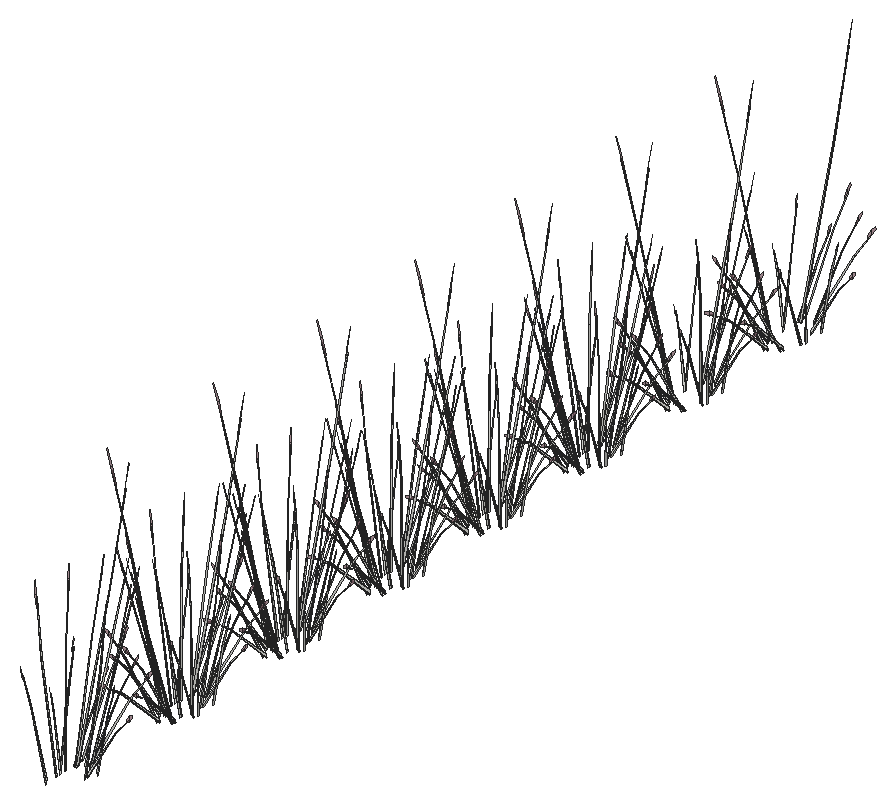
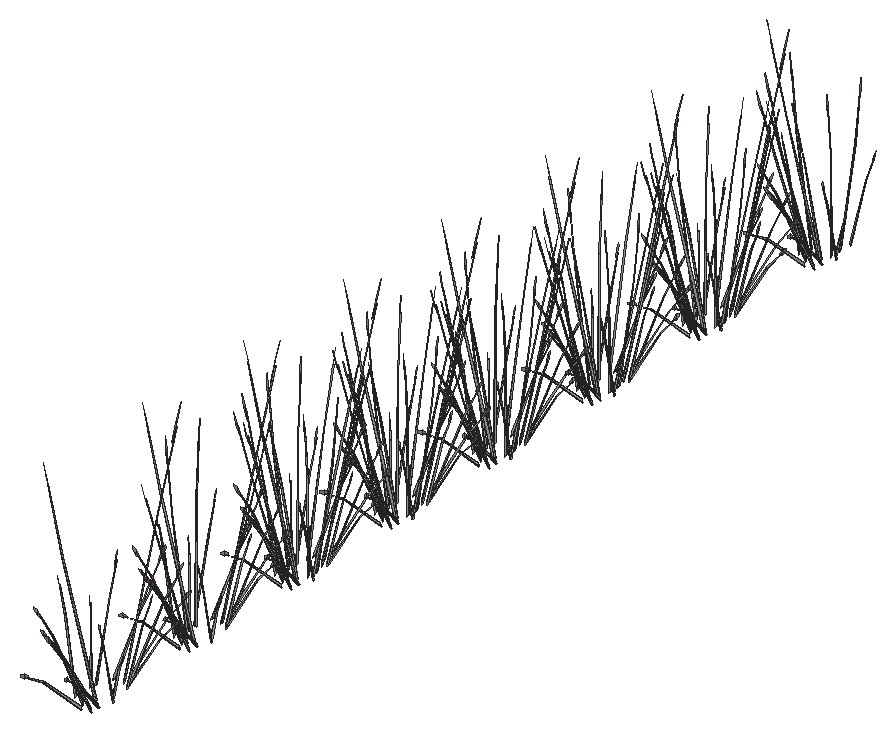
# SketchUp Ruby script. Lengths in inches.
U = 1.inch
M = Sketchup.active_model
def pt(a) = Geom::Point3d.new(a.map { |v| v * U })
def face(e, loops, mat)
  f = e.add_face(loops[0].map { |a| pt(a) })
  loops[1..].each { |l| e.add_face(l.map { |a| pt(a) }).erase! }
  f.material = f.back_material = mat if mat
  f
end
# faces: each face lists its corners as indices into pts; further lists are holes
def faces(e, pts, list, mat = nil) = list.each { |f| face(e, (f[0].is_a?(Array) ? f : [f]).map { |l| l.map { |i| pts[i] } }, mat) }
# xy, xz, yz: faces in a plane at the given z, y or x. An outline is a flat list of corners, or four numbers for a rectangle; further outlines are holes
def ring(l) = l.size == 4 ? [[l[0], l[1]], [l[2], l[1]], [l[2], l[3]], [l[0], l[3]]] : l.each_slice(2).to_a
def flat(e, list, mat, &to3) = list.each { |f| face(e, (f[0].is_a?(Array) ? f : [f]).map { |l| ring(l).map { |u, v| to3.(u, v) } }, mat) }
def xy(e, z, list, mat = nil) = flat(e, list, mat) { |x, y| [x, y, z] }
def xz(e, y, list, mat = nil) = flat(e, list, mat) { |x, z| [x, y, z] }
def yz(e, x, list, mat = nil) = flat(e, list, mat) { |y, z| [x, y, z] }
def lines(e, pts, list) = list.each { |a, b| e.add_line(pt(pts[a]), pt(pts[b])) }
# prism: a flat outline (further loops are holes) pulled along v
def prism(e, loops, v, mat = nil)
  f = face(e, loops, mat); d = Geom::Vector3d.new(v.map { |x| x * U })
  f.pushpull(f.normal.samedirection?(d) ? d.length : -d.length)
end
def box(e, o, s, mat = nil) = prism(e, [[o, [o[0] + s[0], o[1], o[2]], [o[0] + s[0], o[1] + s[1], o[2]], [o[0], o[1] + s[1], o[2]]]], [0, 0, s[2]], mat)
def at(x, y, z, deg = 0) = Geom::Transformation.translation(pt([x, y, z])) * Geom::Transformation.rotation(ORIGIN, Z_AXIS, deg.degrees)
def axes(o, x, y, z) = Geom::Transformation.new([*x, 0, *y, 0, *z, 0, *pt(o).to_a, 1])
def part(name) = M.definitions.add(name)
# library, detail: a bought-in or finely detailed component or shape, given as its bounding box
def library(name, o, s) = part(name).tap { |d| box(d.entities, o, s) }
def detail(e, o, s) = box(e.add_group.entities, o, s)
def put(e, d, t, mat = nil) = e.add_instance(d, t).tap { |i| i.material = mat if mat }
def group(e, t, mat = nil) = e.add_group.tap { |g| g.transformation = t; g.material = mat if mat }.entities
root = M.entities
M.materials.add("LightPink_Translucent").color = [144, 107, 117]
M.materials["LightPink_Translucent"].alpha = 0.75
c1 = part("blade")
p = [[2.15,0.21,22],[0,0.17,0],[0.09,0.45,0],[2.18,0.31,22],[2.29,0.31,22],[0.38,0.45,0],
  [2.48,0.24,33],[2.49,0.24,33],[2.48,0.22,33]]
faces(c1.entities,p,[[0,1,2,3],[4,5,2,3],[6,3,4,7],[8,0,3,6]])
c2 = part("seeds")
p = [[0.3,-0.1,1.38],[-0.01,-0.03,1.59],[-0.01,-0.03,0.03],[0.14,-0.07,-0.07],[0.29,-0.03,3],[0.15,0.01,3.11]]
faces(c2.entities,p,[[0,1,2,3],[1,0,4,5]],"LightPink_Translucent")
c3 = part("blade with seeds")
put(c3.entities,c1,at(0,0,0))
put(c3.entities,c2,axes([2.4,0.25,30.99],[1.5799,-0.05474,1.17369],[-0.12525,1.92788,0.29478],[-0.07173,-0.02425,1.56792]))
put(root,c3,axes([250.48,129.89,2.61],[0.01898,0.06102,1.28742],[-0.09148,0.54852,-0.12165],[-0.09264,0.00397,0.22783]))
put(root,c3,axes([250.44,131.76,2.625],[-0.09401,-0.41691,0.04667],[0.17143,-0.20406,0.3674],[-0.07557,0.04026,0.56022]))
put(root,c3,axes([252.88,132.97,2.625],[0.09401,0.41691,0.04667],[-0.17143,0.20406,0.3674],[0.07557,-0.04026,0.56022]))
put(root,c3,axes([253.29,134.63,2.61],[-0.02314,-0.05353,1.28742],[0.05063,-0.5738,-0.12165],[0.09117,-0.03666,0.22783]))
put(root,c3,axes([250.28,132.3,2.61],[-0.0418,0.07939,1.26972],[0.00356,0.58003,-0.2008],[-0.09581,0.07543,0.10183]))
put(root,c3,axes([252.72,133.76,2.61],[0.05491,-0.01034,1.26972],[0.1506,-0.47504,-0.2008],[0.09767,0.06271,0.10183]))
put(root,c3,axes([250.47,133.1875,2.625],[-0.17571,-0.25715,0.04667],[0.1023,-0.3662,0.3674],[-0.05634,0.11839,0.56022]))
put(root,c3,axes([249.81,132.89,2.61],[0.03267,0.0164,1.28742],[0.10105,0.54025,-0.12165],[-0.06687,0.1418,0.22783]))
put(root,c3,axes([252.58,134.24,2.625],[-0.01289,0.46496,0.04667],[-0.19462,-0.01275,0.3674],[0.07455,0.04865,0.56022]))
put(root,c3,axes([251.78,135.24,2.61],[0.00076,-0.07403,1.28742],[0.21935,-0.3266,-0.12165],[0.07619,0.11658,0.22783]))
put(root,c3,axes([250.82,134.4,2.625],[-0.21034,-0.02849,0.04667],[0.00577,-0.43021,0.3674],[-0.02201,0.1648,0.56022]))
put(root,c3,axes([252.04,135,2.625],[-0.11633,0.38842,0.04667],[-0.16566,-0.22614,0.3674],[0.05356,0.12453,0.56022]))
put(root,c3,axes([251.39,135.06,2.625],[-0.1886,0.20781,0.04667],[-0.09231,-0.37894,0.3674],[0.01821,0.16704,0.56022]))
put(root,c3,axes([250.29,134.46,2.61],[-0.00636,0.121,1.26972],[0.18056,0.42094,-0.2008],[-0.04727,0.19906,0.10183]))
put(root,c3,axes([250.86,134.19,3.11],[0.2813,0.0303,-0.09797],[-0.00769,0.57361,-0.54375],[-0.01954,0.22092,0.82622]))
put(root,c3,axes([250.27,135.71,2.61],[0.02904,-0.03692,1.28742],[0.24001,0.24555,-0.12165],[-0.00564,0.20445,0.22783]))
put(root,c3,axes([251.32,135.96,2.61],[0.03244,0.09846,1.26972],[0.26183,0.03868,-0.2008],[0.02633,0.21715,0.10183]))
put(root,c3,axes([251.55,146.22,2.61],[-0.03915,-0.08573,1.26972],[-0.26126,0.05435,-0.2008],[-0.0417,-0.20505,0.10183]))
put(root,c3,axes([252.72,147.27,2.61],[-0.00247,-0.12169,1.26972],[-0.20868,-0.35171,-0.2008],[0.03226,-0.2132,0.10183]))
put(root,c3,axes([252.66,146.83,2.61],[-0.02599,0.0467,1.28742],[-0.25468,-0.15757,-0.12165],[-0.00922,-0.20381,0.22783]))
put(root,c3,axes([251.28,145.9375,2.61],[-0.00478,0.07329,1.28742],[-0.23551,0.26599,-0.12165],[-0.0693,-0.13596,0.22783]))
put(root,c3,axes([251.9375,147.3125,2.625],[0.1886,-0.20781,0.04667],[0.09231,0.37894,0.3674],[-0.01821,-0.16704,0.56022]))
put(root,c3,axes([251.29,147.37,2.625],[0.11633,-0.38842,0.04667],[0.16566,0.22614,0.3674],[-0.05356,-0.12453,0.56022]))
put(root,c3,axes([251.34,147.33,3.13],[-0.17082,0.58618,-0.09885],[-0.24738,-0.33771,-0.54865],[-0.08599,-0.16561,0.83366]))
put(root,c3,axes([252.51,147.98,2.625],[0.21034,0.02849,0.04667],[-0.00577,0.43021,0.3674],[0.02201,-0.1648,0.56022]))
put(root,c3,axes([250.6875,147.16,2.61],[-0.05507,-0.00432,1.26972],[-0.17533,0.4316,-0.2008],[-0.09355,-0.08819,0.10183]))
put(root,c3,axes([253.35,149.16,2.61],[-0.03343,-0.00464,1.28742],[-0.13883,-0.49759,-0.12165],[0.05575,-0.16361,0.22783]))
put(root,c3,axes([250.75,148.14,2.625],[0.01289,-0.46496,0.04667],[0.19462,0.01275,0.3674],[-0.07455,-0.04865,0.56022]))
put(root,c3,axes([252.86,149.19,2.625],[0.17571,0.25715,0.04667],[-0.1023,0.3662,0.3674],[0.05634,-0.11839,0.56022]))
put(root,c3,axes([253.48,149.76,2.61],[0.03552,-0.09314,1.26972],[-0.04546,-0.57131,-0.2008],[0.08912,-0.10832,0.10183]))
put(root,c3,axes([250.48,147.53,2.61],[0.01898,0.06102,1.28742],[-0.09148,0.54852,-0.12165],[-0.09264,0.00397,0.22783]))
put(root,c3,axes([250.44,149.4,2.625],[-0.09401,-0.41691,0.04667],[0.17143,-0.20406,0.3674],[-0.07557,0.04026,0.56022]))
put(root,c3,axes([252.88,150.61,2.625],[0.09401,0.41691,0.04667],[-0.17143,0.20406,0.3674],[0.07557,-0.04026,0.56022]))
put(root,c3,axes([253.29,152.27,2.61],[-0.02314,-0.05353,1.28742],[0.05063,-0.5738,-0.12165],[0.09117,-0.03666,0.22783]))
put(root,c3,axes([250.28,149.94,2.61],[-0.0418,0.07939,1.26972],[0.00356,0.58003,-0.2008],[-0.09581,0.07543,0.10183]))
put(root,c3,axes([252.72,151.4,2.61],[0.05491,-0.01034,1.26972],[0.1506,-0.47504,-0.2008],[0.09767,0.06271,0.10183]))
put(root,c3,axes([250.47,150.83,2.625],[-0.17571,-0.25715,0.04667],[0.1023,-0.3662,0.3674],[-0.05634,0.11839,0.56022]))
put(root,c3,axes([249.81,150.53,2.61],[0.03267,0.0164,1.28742],[0.10105,0.54025,-0.12165],[-0.06687,0.1418,0.22783]))
put(root,c3,axes([252.58,151.88,2.625],[-0.01289,0.46496,0.04667],[-0.19462,-0.01275,0.3674],[0.07455,0.04865,0.56022]))
put(root,c3,axes([251.78,152.89,2.61],[0.00076,-0.07403,1.28742],[0.21935,-0.3266,-0.12165],[0.07619,0.11658,0.22783]))
put(root,c3,axes([250.82,152.04,2.625],[-0.21034,-0.02849,0.04667],[0.00577,-0.43021,0.3674],[-0.02201,0.1648,0.56022]))
put(root,c3,axes([252.04,152.64,2.625],[-0.11633,0.38842,0.04667],[-0.16566,-0.22614,0.3674],[0.05356,0.12453,0.56022]))
put(root,c3,axes([251.39,152.7,2.625],[-0.1886,0.20781,0.04667],[-0.09231,-0.37894,0.3674],[0.01821,0.16704,0.56022]))
put(root,c3,axes([250.29,152.11,2.61],[-0.00636,0.121,1.26972],[0.18056,0.42094,-0.2008],[-0.04727,0.19906,0.10183]))
put(root,c3,axes([250.86,151.83,3.11],[0.2813,0.0303,-0.09797],[-0.00769,0.57361,-0.54375],[-0.01954,0.22092,0.82622]))
put(root,c3,axes([250.27,153.35,2.61],[0.02904,-0.03692,1.28742],[0.24001,0.24555,-0.12165],[-0.00564,0.20445,0.22783]))
put(root,c3,axes([251.32,153.6,2.61],[0.03244,0.09846,1.26972],[0.26183,0.03868,-0.2008],[0.02633,0.21715,0.10183]))
put(root,c3,axes([251.55,162.49,2.61],[-0.03915,-0.08573,1.26972],[-0.26126,0.05435,-0.2008],[-0.0417,-0.20505,0.10183]))
put(root,c3,axes([252.72,163.54,2.61],[-0.00247,-0.12169,1.26972],[-0.20868,-0.35171,-0.2008],[0.03226,-0.2132,0.10183]))
put(root,c3,axes([252.66,163.1,2.61],[-0.02599,0.0467,1.28742],[-0.25468,-0.15757,-0.12165],[-0.00922,-0.20381,0.22783]))
put(root,c3,axes([251.28,162.21,2.61],[-0.00478,0.07329,1.28742],[-0.23551,0.26599,-0.12165],[-0.0693,-0.13596,0.22783]))
put(root,c3,axes([251.9375,163.58,2.625],[0.1886,-0.20781,0.04667],[0.09231,0.37894,0.3674],[-0.01821,-0.16704,0.56022]))
put(root,c3,axes([251.29,163.64,2.625],[0.11633,-0.38842,0.04667],[0.16566,0.22614,0.3674],[-0.05356,-0.12453,0.56022]))
put(root,c3,axes([251.34,163.6,3.13],[-0.17082,0.58618,-0.09885],[-0.24738,-0.33771,-0.54865],[-0.08599,-0.16561,0.83366]))
put(root,c3,axes([252.51,164.25,2.625],[0.21034,0.02849,0.04667],[-0.00577,0.43021,0.3674],[0.02201,-0.1648,0.56022]))
put(root,c3,axes([250.6875,163.43,2.61],[-0.05507,-0.00432,1.26972],[-0.17533,0.4316,-0.2008],[-0.09355,-0.08819,0.10183]))
put(root,c3,axes([253.35,165.43,2.61],[-0.03343,-0.00464,1.28742],[-0.13883,-0.49759,-0.12165],[0.05575,-0.16361,0.22783]))
put(root,c3,axes([250.75,164.41,2.625],[0.01289,-0.46496,0.04667],[0.19462,0.01275,0.3674],[-0.07455,-0.04865,0.56022]))
put(root,c3,axes([252.86,165.46,2.625],[0.17571,0.25715,0.04667],[-0.1023,0.3662,0.3674],[0.05634,-0.11839,0.56022]))
put(root,c3,axes([253.48,166.03,2.61],[0.03552,-0.09314,1.26972],[-0.04546,-0.57131,-0.2008],[0.08912,-0.10832,0.10183]))
put(root,c3,axes([250.48,163.8,2.61],[0.01898,0.06102,1.28742],[-0.09148,0.54852,-0.12165],[-0.09264,0.00397,0.22783]))
put(root,c3,axes([250.44,165.67,2.625],[-0.09401,-0.41691,0.04667],[0.17143,-0.20406,0.3674],[-0.07557,0.04026,0.56022]))
put(root,c3,axes([252.88,166.88,2.625],[0.09401,0.41691,0.04667],[-0.17143,0.20406,0.3674],[0.07557,-0.04026,0.56022]))
put(root,c3,axes([253.29,168.54,2.61],[-0.02314,-0.05353,1.28742],[0.05063,-0.5738,-0.12165],[0.09117,-0.03666,0.22783]))
put(root,c3,axes([250.28,166.21,2.61],[-0.0418,0.07939,1.26972],[0.00356,0.58003,-0.2008],[-0.09581,0.07543,0.10183]))
put(root,c3,axes([252.72,167.67,2.61],[0.05491,-0.01034,1.26972],[0.1506,-0.47504,-0.2008],[0.09767,0.06271,0.10183]))
put(root,c3,axes([250.47,167.1,2.625],[-0.17571,-0.25715,0.04667],[0.1023,-0.3662,0.3674],[-0.05634,0.11839,0.56022]))
put(root,c3,axes([249.81,166.8,2.61],[0.03267,0.0164,1.28742],[0.10105,0.54025,-0.12165],[-0.06687,0.1418,0.22783]))
put(root,c3,axes([252.58,168.15,2.625],[-0.01289,0.46496,0.04667],[-0.19462,-0.01275,0.3674],[0.07455,0.04865,0.56022]))
put(root,c3,axes([251.78,169.16,2.61],[0.00076,-0.07403,1.28742],[0.21935,-0.3266,-0.12165],[0.07619,0.11658,0.22783]))
put(root,c3,axes([250.82,168.31,2.625],[-0.21034,-0.02849,0.04667],[0.00577,-0.43021,0.3674],[-0.02201,0.1648,0.56022]))
put(root,c3,axes([252.04,168.91,2.625],[-0.11633,0.38842,0.04667],[-0.16566,-0.22614,0.3674],[0.05356,0.12453,0.56022]))
put(root,c3,axes([251.39,168.97,2.625],[-0.1886,0.20781,0.04667],[-0.09231,-0.37894,0.3674],[0.01821,0.16704,0.56022]))
put(root,c3,axes([250.29,168.38,2.61],[-0.00636,0.121,1.26972],[0.18056,0.42094,-0.2008],[-0.04727,0.19906,0.10183]))
put(root,c3,axes([250.86,168.1,3.11],[0.2813,0.0303,-0.09797],[-0.00769,0.57361,-0.54375],[-0.01954,0.22092,0.82622]))
put(root,c3,axes([250.27,169.62,2.61],[0.02904,-0.03692,1.28742],[0.24001,0.24555,-0.12165],[-0.00564,0.20445,0.22783]))
put(root,c3,axes([251.32,169.875,2.61],[0.03244,0.09846,1.26972],[0.26183,0.03868,-0.2008],[0.02633,0.21715,0.10183]))
put(root,c3,axes([251.55,178.34,2.61],[-0.03915,-0.08573,1.26972],[-0.26126,0.05435,-0.2008],[-0.0417,-0.20505,0.10183]))
put(root,c3,axes([252.72,179.39,2.61],[-0.00247,-0.12169,1.26972],[-0.20868,-0.35171,-0.2008],[0.03226,-0.2132,0.10183]))
put(root,c3,axes([252.66,178.95,2.61],[-0.02599,0.0467,1.28742],[-0.25468,-0.15757,-0.12165],[-0.00922,-0.20381,0.22783]))
put(root,c3,axes([251.28,178.06,2.61],[-0.00478,0.07329,1.28742],[-0.23551,0.26599,-0.12165],[-0.0693,-0.13596,0.22783]))
put(root,c3,axes([251.9375,179.43,2.625],[0.1886,-0.20781,0.04667],[0.09231,0.37894,0.3674],[-0.01821,-0.16704,0.56022]))
put(root,c3,axes([251.29,179.49,2.625],[0.11633,-0.38842,0.04667],[0.16566,0.22614,0.3674],[-0.05356,-0.12453,0.56022]))
put(root,c3,axes([251.34,179.45,3.13],[-0.17082,0.58618,-0.09885],[-0.24738,-0.33771,-0.54865],[-0.08599,-0.16561,0.83366]))
put(root,c3,axes([252.51,180.1,2.625],[0.21034,0.02849,0.04667],[-0.00577,0.43021,0.3674],[0.02201,-0.1648,0.56022]))
put(root,c3,axes([250.6875,179.28,2.61],[-0.05507,-0.00432,1.26972],[-0.17533,0.4316,-0.2008],[-0.09355,-0.08819,0.10183]))
put(root,c3,axes([253.35,181.28,2.61],[-0.03343,-0.00464,1.28742],[-0.13883,-0.49759,-0.12165],[0.05575,-0.16361,0.22783]))
put(root,c3,axes([250.75,180.26,2.625],[0.01289,-0.46496,0.04667],[0.19462,0.01275,0.3674],[-0.07455,-0.04865,0.56022]))
put(root,c3,axes([252.86,181.31,2.625],[0.17571,0.25715,0.04667],[-0.1023,0.3662,0.3674],[0.05634,-0.11839,0.56022]))
put(root,c3,axes([253.48,181.88,2.61],[0.03552,-0.09314,1.26972],[-0.04546,-0.57131,-0.2008],[0.08912,-0.10832,0.10183]))
put(root,c3,axes([250.48,179.65,2.61],[0.01898,0.06102,1.28742],[-0.09148,0.54852,-0.12165],[-0.09264,0.00397,0.22783]))
put(root,c3,axes([250.44,181.52,2.625],[-0.09401,-0.41691,0.04667],[0.17143,-0.20406,0.3674],[-0.07557,0.04026,0.56022]))
put(root,c3,axes([252.88,182.73,2.625],[0.09401,0.41691,0.04667],[-0.17143,0.20406,0.3674],[0.07557,-0.04026,0.56022]))
put(root,c3,axes([253.29,184.39,2.61],[-0.02314,-0.05353,1.28742],[0.05063,-0.5738,-0.12165],[0.09117,-0.03666,0.22783]))
put(root,c3,axes([250.28,182.0625,2.61],[-0.0418,0.07939,1.26972],[0.00356,0.58003,-0.2008],[-0.09581,0.07543,0.10183]))
put(root,c3,axes([252.72,183.52,2.61],[0.05491,-0.01034,1.26972],[0.1506,-0.47504,-0.2008],[0.09767,0.06271,0.10183]))
put(root,c3,axes([250.47,182.95,2.625],[-0.17571,-0.25715,0.04667],[0.1023,-0.3662,0.3674],[-0.05634,0.11839,0.56022]))
put(root,c3,axes([249.81,182.65,2.61],[0.03267,0.0164,1.28742],[0.10105,0.54025,-0.12165],[-0.06687,0.1418,0.22783]))
put(root,c3,axes([252.58,184,2.625],[-0.01289,0.46496,0.04667],[-0.19462,-0.01275,0.3674],[0.07455,0.04865,0.56022]))
put(root,c3,axes([251.78,185.01,2.61],[0.00076,-0.07403,1.28742],[0.21935,-0.3266,-0.12165],[0.07619,0.11658,0.22783]))
put(root,c3,axes([250.82,184.16,2.625],[-0.21034,-0.02849,0.04667],[0.00577,-0.43021,0.3674],[-0.02201,0.1648,0.56022]))
put(root,c3,axes([252.04,184.77,2.625],[-0.11633,0.38842,0.04667],[-0.16566,-0.22614,0.3674],[0.05356,0.12453,0.56022]))
put(root,c3,axes([251.39,184.82,2.625],[-0.1886,0.20781,0.04667],[-0.09231,-0.37894,0.3674],[0.01821,0.16704,0.56022]))
put(root,c3,axes([250.29,184.23,2.61],[-0.00636,0.121,1.26972],[0.18056,0.42094,-0.2008],[-0.04727,0.19906,0.10183]))
put(root,c3,axes([250.86,183.96,3.11],[0.2813,0.0303,-0.09797],[-0.00769,0.57361,-0.54375],[-0.01954,0.22092,0.82622]))
put(root,c3,axes([250.27,185.47,2.61],[0.02904,-0.03692,1.28742],[0.24001,0.24555,-0.12165],[-0.00564,0.20445,0.22783]))
put(root,c3,axes([251.55,193.33,2.61],[-0.03915,-0.08573,1.26972],[-0.26126,0.05435,-0.2008],[-0.0417,-0.20505,0.10183]))
put(root,c3,axes([251.32,185.73,2.61],[0.03244,0.09846,1.26972],[0.26183,0.03868,-0.2008],[0.02633,0.21715,0.10183]))
put(root,c3,axes([252.72,194.375,2.61],[-0.00247,-0.12169,1.26972],[-0.20868,-0.35171,-0.2008],[0.03226,-0.2132,0.10183]))
put(root,c3,axes([252.66,193.94,2.61],[-0.02599,0.0467,1.28742],[-0.25468,-0.15757,-0.12165],[-0.00922,-0.20381,0.22783]))
put(root,c3,axes([251.28,193.04,2.61],[-0.00478,0.07329,1.28742],[-0.23551,0.26599,-0.12165],[-0.0693,-0.13596,0.22783]))
put(root,c3,axes([251.9375,194.42,2.625],[0.1886,-0.20781,0.04667],[0.09231,0.37894,0.3674],[-0.01821,-0.16704,0.56022]))
put(root,c3,axes([251.29,194.48,2.625],[0.11633,-0.38842,0.04667],[0.16566,0.22614,0.3674],[-0.05356,-0.12453,0.56022]))
put(root,c3,axes([251.34,194.4375,3.13],[-0.17082,0.58618,-0.09885],[-0.24738,-0.33771,-0.54865],[-0.08599,-0.16561,0.83366]))
put(root,c3,axes([252.51,195.08,2.625],[0.21034,0.02849,0.04667],[-0.00577,0.43021,0.3674],[0.02201,-0.1648,0.56022]))
put(root,c3,axes([250.6875,194.27,2.61],[-0.05507,-0.00432,1.26972],[-0.17533,0.4316,-0.2008],[-0.09355,-0.08819,0.10183]))
put(root,c3,axes([253.35,196.27,2.61],[-0.03343,-0.00464,1.28742],[-0.13883,-0.49759,-0.12165],[0.05575,-0.16361,0.22783]))
put(root,c3,axes([250.75,195.24,2.625],[0.01289,-0.46496,0.04667],[0.19462,0.01275,0.3674],[-0.07455,-0.04865,0.56022]))
put(root,c3,axes([252.86,196.29,2.625],[0.17571,0.25715,0.04667],[-0.1023,0.3662,0.3674],[0.05634,-0.11839,0.56022]))
put(root,c3,axes([253.48,196.87,2.61],[0.03552,-0.09314,1.26972],[-0.04546,-0.57131,-0.2008],[0.08912,-0.10832,0.10183]))
put(root,c3,axes([250.48,194.64,2.61],[0.01898,0.06102,1.28742],[-0.09148,0.54852,-0.12165],[-0.09264,0.00397,0.22783]))
put(root,c3,axes([250.44,196.51,2.625],[-0.09401,-0.41691,0.04667],[0.17143,-0.20406,0.3674],[-0.07557,0.04026,0.56022]))
put(root,c3,axes([252.88,197.72,2.625],[0.09401,0.41691,0.04667],[-0.17143,0.20406,0.3674],[0.07557,-0.04026,0.56022]))
put(root,c3,axes([253.29,199.38,2.61],[-0.02314,-0.05353,1.28742],[0.05063,-0.5738,-0.12165],[0.09117,-0.03666,0.22783]))
put(root,c3,axes([250.28,197.05,2.61],[-0.0418,0.07939,1.26972],[0.00356,0.58003,-0.2008],[-0.09581,0.07543,0.10183]))
put(root,c3,axes([252.72,198.51,2.61],[0.05491,-0.01034,1.26972],[0.1506,-0.47504,-0.2008],[0.09767,0.06271,0.10183]))
put(root,c3,axes([250.47,197.9375,2.625],[-0.17571,-0.25715,0.04667],[0.1023,-0.3662,0.3674],[-0.05634,0.11839,0.56022]))
put(root,c3,axes([249.81,197.64,2.61],[0.03267,0.0164,1.28742],[0.10105,0.54025,-0.12165],[-0.06687,0.1418,0.22783]))
put(root,c3,axes([252.58,198.99,2.625],[-0.01289,0.46496,0.04667],[-0.19462,-0.01275,0.3674],[0.07455,0.04865,0.56022]))
put(root,c3,axes([251.78,199.99,2.61],[0.00076,-0.07403,1.28742],[0.21935,-0.3266,-0.12165],[0.07619,0.11658,0.22783]))
put(root,c3,axes([250.82,199.15,2.625],[-0.21034,-0.02849,0.04667],[0.00577,-0.43021,0.3674],[-0.02201,0.1648,0.56022]))
put(root,c3,axes([252.04,199.75,2.625],[-0.11633,0.38842,0.04667],[-0.16566,-0.22614,0.3674],[0.05356,0.12453,0.56022]))
put(root,c3,axes([251.39,199.81,2.625],[-0.1886,0.20781,0.04667],[-0.09231,-0.37894,0.3674],[0.01821,0.16704,0.56022]))
put(root,c3,axes([250.29,199.21,2.61],[-0.00636,0.121,1.26972],[0.18056,0.42094,-0.2008],[-0.04727,0.19906,0.10183]))
put(root,c3,axes([250.86,198.94,3.11],[0.2813,0.0303,-0.09797],[-0.00769,0.57361,-0.54375],[-0.01954,0.22092,0.82622]))
put(root,c3,axes([250.27,200.46,2.61],[0.02904,-0.03692,1.28742],[0.24001,0.24555,-0.12165],[-0.00564,0.20445,0.22783]))
put(root,c3,axes([251.55,208.58,2.61],[-0.03915,-0.08573,1.26972],[-0.26126,0.05435,-0.2008],[-0.0417,-0.20505,0.10183]))
put(root,c3,axes([251.32,200.71,2.61],[0.03244,0.09846,1.26972],[0.26183,0.03868,-0.2008],[0.02633,0.21715,0.10183]))
put(root,c3,axes([252.72,209.63,2.61],[-0.00247,-0.12169,1.26972],[-0.20868,-0.35171,-0.2008],[0.03226,-0.2132,0.10183]))
put(root,c3,axes([252.66,209.19,2.61],[-0.02599,0.0467,1.28742],[-0.25468,-0.15757,-0.12165],[-0.00922,-0.20381,0.22783]))
put(root,c3,axes([251.28,208.3,2.61],[-0.00478,0.07329,1.28742],[-0.23551,0.26599,-0.12165],[-0.0693,-0.13596,0.22783]))
put(root,c3,axes([251.9375,209.67,2.625],[0.1886,-0.20781,0.04667],[0.09231,0.37894,0.3674],[-0.01821,-0.16704,0.56022]))
put(root,c3,axes([251.29,209.73,2.625],[0.11633,-0.38842,0.04667],[0.16566,0.22614,0.3674],[-0.05356,-0.12453,0.56022]))
put(root,c3,axes([251.34,209.69,3.13],[-0.17082,0.58618,-0.09885],[-0.24738,-0.33771,-0.54865],[-0.08599,-0.16561,0.83366]))
put(root,c3,axes([252.51,210.34,2.625],[0.21034,0.02849,0.04667],[-0.00577,0.43021,0.3674],[0.02201,-0.1648,0.56022]))
put(root,c3,axes([250.6875,209.52,2.61],[-0.05507,-0.00432,1.26972],[-0.17533,0.4316,-0.2008],[-0.09355,-0.08819,0.10183]))
put(root,c3,axes([253.35,211.52,2.61],[-0.03343,-0.00464,1.28742],[-0.13883,-0.49759,-0.12165],[0.05575,-0.16361,0.22783]))
put(root,c3,axes([250.75,210.5,2.625],[0.01289,-0.46496,0.04667],[0.19462,0.01275,0.3674],[-0.07455,-0.04865,0.56022]))
put(root,c3,axes([252.86,211.55,2.625],[0.17571,0.25715,0.04667],[-0.1023,0.3662,0.3674],[0.05634,-0.11839,0.56022]))
put(root,c3,axes([253.48,212.12,2.61],[0.03552,-0.09314,1.26972],[-0.04546,-0.57131,-0.2008],[0.08912,-0.10832,0.10183]))
put(root,c3,axes([250.48,209.89,2.61],[0.01898,0.06102,1.28742],[-0.09148,0.54852,-0.12165],[-0.09264,0.00397,0.22783]))
put(root,c3,axes([250.44,211.76,2.625],[-0.09401,-0.41691,0.04667],[0.17143,-0.20406,0.3674],[-0.07557,0.04026,0.56022]))
put(root,c3,axes([252.88,212.97,2.625],[0.09401,0.41691,0.04667],[-0.17143,0.20406,0.3674],[0.07557,-0.04026,0.56022]))
put(root,c3,axes([253.29,214.63,2.61],[-0.02314,-0.05353,1.28742],[0.05063,-0.5738,-0.12165],[0.09117,-0.03666,0.22783]))
put(root,c3,axes([250.28,212.3,2.61],[-0.0418,0.07939,1.26972],[0.00356,0.58003,-0.2008],[-0.09581,0.07543,0.10183]))
put(root,c3,axes([252.72,213.76,2.61],[0.05491,-0.01034,1.26972],[0.1506,-0.47504,-0.2008],[0.09767,0.06271,0.10183]))
put(root,c3,axes([250.47,213.19,2.625],[-0.17571,-0.25715,0.04667],[0.1023,-0.3662,0.3674],[-0.05634,0.11839,0.56022]))
put(root,c3,axes([249.81,212.89,2.61],[0.03267,0.0164,1.28742],[0.10105,0.54025,-0.12165],[-0.06687,0.1418,0.22783]))
put(root,c3,axes([252.58,214.24,2.625],[-0.01289,0.46496,0.04667],[-0.19462,-0.01275,0.3674],[0.07455,0.04865,0.56022]))
put(root,c3,axes([251.78,215.25,2.61],[0.00076,-0.07403,1.28742],[0.21935,-0.3266,-0.12165],[0.07619,0.11658,0.22783]))
put(root,c3,axes([250.82,214.4,2.625],[-0.21034,-0.02849,0.04667],[0.00577,-0.43021,0.3674],[-0.02201,0.1648,0.56022]))
put(root,c3,axes([252.04,215,2.625],[-0.11633,0.38842,0.04667],[-0.16566,-0.22614,0.3674],[0.05356,0.12453,0.56022]))
put(root,c3,axes([251.39,215.0625,2.625],[-0.1886,0.20781,0.04667],[-0.09231,-0.37894,0.3674],[0.01821,0.16704,0.56022]))
put(root,c3,axes([250.29,214.47,2.61],[-0.00636,0.121,1.26972],[0.18056,0.42094,-0.2008],[-0.04727,0.19906,0.10183]))
put(root,c3,axes([250.86,214.19,3.11],[0.2813,0.0303,-0.09797],[-0.00769,0.57361,-0.54375],[-0.01954,0.22092,0.82622]))
put(root,c3,axes([250.27,215.71,2.61],[0.02904,-0.03692,1.28742],[0.24001,0.24555,-0.12165],[-0.00564,0.20445,0.22783]))
put(root,c3,axes([251.32,215.96,2.61],[0.03244,0.09846,1.26972],[0.26183,0.03868,-0.2008],[0.02633,0.21715,0.10183]))
put(root,c3,axes([251.55,224.09,2.61],[-0.03915,-0.08573,1.26972],[-0.26126,0.05435,-0.2008],[-0.0417,-0.20505,0.10183]))
put(root,c3,axes([252.72,225.14,2.61],[-0.00247,-0.12169,1.26972],[-0.20868,-0.35171,-0.2008],[0.03226,-0.2132,0.10183]))
put(root,c3,axes([252.66,224.7,2.61],[-0.02599,0.0467,1.28742],[-0.25468,-0.15757,-0.12165],[-0.00922,-0.20381,0.22783]))
put(root,c3,axes([251.28,223.81,2.61],[-0.00478,0.07329,1.28742],[-0.23551,0.26599,-0.12165],[-0.0693,-0.13596,0.22783]))
put(root,c3,axes([251.29,225.24,2.625],[0.11633,-0.38842,0.04667],[0.16566,0.22614,0.3674],[-0.05356,-0.12453,0.56022]))
put(root,c3,axes([251.34,225.2,3.13],[-0.17082,0.58618,-0.09885],[-0.24738,-0.33771,-0.54865],[-0.08599,-0.16561,0.83366]))
put(root,c3,axes([250.6875,225.03,2.61],[-0.05507,-0.00432,1.26972],[-0.17533,0.4316,-0.2008],[-0.09355,-0.08819,0.10183]))
put(root,c3,axes([253.35,227.03,2.61],[-0.03343,-0.00464,1.28742],[-0.13883,-0.49759,-0.12165],[0.05575,-0.16361,0.22783]))
put(root,c3,axes([252.86,227.05,2.625],[0.17571,0.25715,0.04667],[-0.1023,0.3662,0.3674],[0.05634,-0.11839,0.56022]))
put(root,c3,axes([253.48,227.63,2.61],[0.03552,-0.09314,1.26972],[-0.04546,-0.57131,-0.2008],[0.08912,-0.10832,0.10183]))
put(root,c3,axes([250.48,225.4,2.61],[0.01898,0.06102,1.28742],[-0.09148,0.54852,-0.12165],[-0.09264,0.00397,0.22783]))
put(root,c3,axes([252.88,228.48,2.625],[0.09401,0.41691,0.04667],[-0.17143,0.20406,0.3674],[0.07557,-0.04026,0.56022]))
put(root,c3,axes([253.29,230.14,2.61],[-0.02314,-0.05353,1.28742],[0.05063,-0.5738,-0.12165],[0.09117,-0.03666,0.22783]))
put(root,c3,axes([250.28,227.8125,2.61],[-0.0418,0.07939,1.26972],[0.00356,0.58003,-0.2008],[-0.09581,0.07543,0.10183]))
put(root,c3,axes([252.72,229.27,2.61],[0.05491,-0.01034,1.26972],[0.1506,-0.47504,-0.2008],[0.09767,0.06271,0.10183]))
put(root,c3,axes([249.81,228.4,2.61],[0.03267,0.0164,1.28742],[0.10105,0.54025,-0.12165],[-0.06687,0.1418,0.22783]))
put(root,c3,axes([251.78,230.76,2.61],[0.00076,-0.07403,1.28742],[0.21935,-0.3266,-0.12165],[0.07619,0.11658,0.22783]))
put(root,c3,axes([251.39,230.57,2.625],[-0.1886,0.20781,0.04667],[-0.09231,-0.37894,0.3674],[0.01821,0.16704,0.56022]))
put(root,c3,axes([250.29,229.98,2.61],[-0.00636,0.121,1.26972],[0.18056,0.42094,-0.2008],[-0.04727,0.19906,0.10183]))
put(root,c3,axes([250.86,229.7,3.11],[0.2813,0.0303,-0.09797],[-0.00769,0.57361,-0.54375],[-0.01954,0.22092,0.82622]))
put(root,c3,axes([250.27,231.22,2.61],[0.02904,-0.03692,1.28742],[0.24001,0.24555,-0.12165],[-0.00564,0.20445,0.22783]))
put(root,c3,axes([251.55,239.17,2.61],[-0.03915,-0.08573,1.26972],[-0.26126,0.05435,-0.2008],[-0.0417,-0.20505,0.10183]))
put(root,c3,axes([251.32,231.47,2.61],[0.03244,0.09846,1.26972],[0.26183,0.03868,-0.2008],[0.02633,0.21715,0.10183]))
put(root,c3,axes([252.72,240.22,2.61],[-0.00247,-0.12169,1.26972],[-0.20868,-0.35171,-0.2008],[0.03226,-0.2132,0.10183]))
put(root,c3,axes([252.66,239.79,2.61],[-0.02599,0.0467,1.28742],[-0.25468,-0.15757,-0.12165],[-0.00922,-0.20381,0.22783]))
put(root,c3,axes([251.28,238.89,2.61],[-0.00478,0.07329,1.28742],[-0.23551,0.26599,-0.12165],[-0.0693,-0.13596,0.22783]))
put(root,c3,axes([251.34,240.28,3.13],[-0.17082,0.58618,-0.09885],[-0.24738,-0.33771,-0.54865],[-0.08599,-0.16561,0.83366]))
put(root,c3,axes([250.6875,240.12,2.61],[-0.05507,-0.00432,1.26972],[-0.17533,0.4316,-0.2008],[-0.09355,-0.08819,0.10183]))
put(root,c3,axes([253.35,242.12,2.61],[-0.03343,-0.00464,1.28742],[-0.13883,-0.49759,-0.12165],[0.05575,-0.16361,0.22783]))
put(root,c3,axes([253.48,242.71,2.61],[0.03552,-0.09314,1.26972],[-0.04546,-0.57131,-0.2008],[0.08912,-0.10832,0.10183]))
put(root,c3,axes([250.48,240.48,2.61],[0.01898,0.06102,1.28742],[-0.09148,0.54852,-0.12165],[-0.09264,0.00397,0.22783]))
put(root,c3,axes([253.29,245.22,2.61],[-0.02314,-0.05353,1.28742],[0.05063,-0.5738,-0.12165],[0.09117,-0.03666,0.22783]))
put(root,c3,axes([250.28,242.9,2.61],[-0.0418,0.07939,1.26972],[0.00356,0.58003,-0.2008],[-0.09581,0.07543,0.10183]))
put(root,c3,axes([252.72,244.36,2.61],[0.05491,-0.01034,1.26972],[0.1506,-0.47504,-0.2008],[0.09767,0.06271,0.10183]))
put(root,c3,axes([249.81,243.48,2.61],[0.03267,0.0164,1.28742],[0.10105,0.54025,-0.12165],[-0.06687,0.1418,0.22783]))
put(root,c3,axes([251.78,245.84,2.61],[0.00076,-0.07403,1.28742],[0.21935,-0.3266,-0.12165],[0.07619,0.11658,0.22783]))
put(root,c3,axes([250.29,245.0625,2.61],[-0.00636,0.121,1.26972],[0.18056,0.42094,-0.2008],[-0.04727,0.19906,0.10183]))
put(root,c3,axes([250.86,244.79,3.11],[0.2813,0.0303,-0.09797],[-0.00769,0.57361,-0.54375],[-0.01954,0.22092,0.82622]))
put(root,c3,axes([250.27,246.3,2.61],[0.02904,-0.03692,1.28742],[0.24001,0.24555,-0.12165],[-0.00564,0.20445,0.22783]))
put(root,c3,axes([251.32,246.56,2.61],[0.03244,0.09846,1.26972],[0.26183,0.03868,-0.2008],[0.02633,0.21715,0.10183]))
